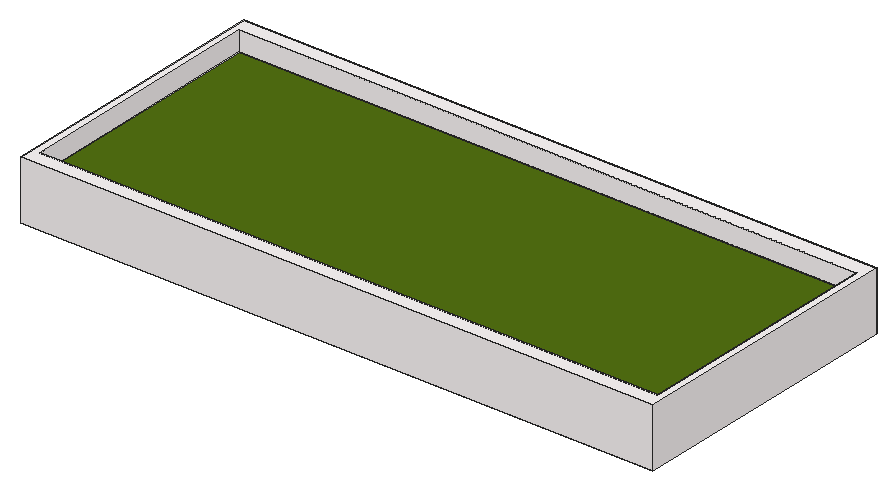
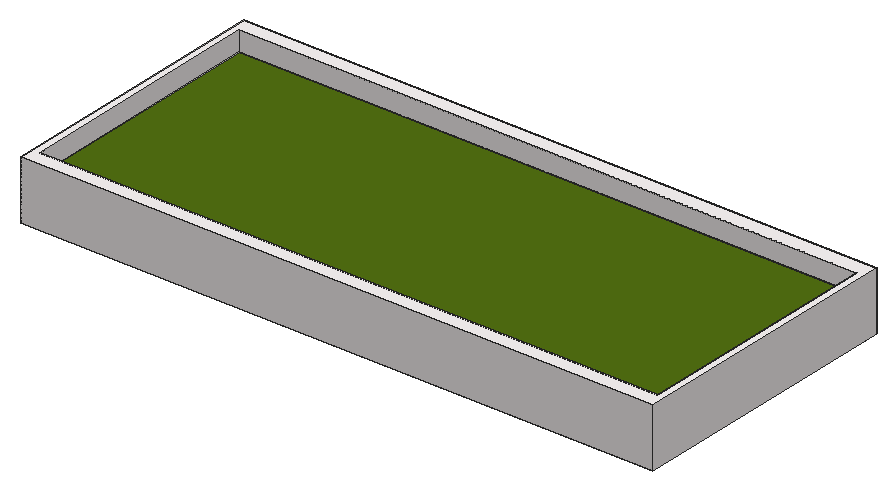
# SketchUp Ruby script. Lengths in inches.
U = 1.inch
M = Sketchup.active_model
def pt(a) = Geom::Point3d.new(a.map { |v| v * U })
def face(e, loops, mat)
  f = e.add_face(loops[0].map { |a| pt(a) })
  loops[1..].each { |l| e.add_face(l.map { |a| pt(a) }).erase! }
  f.material = f.back_material = mat if mat
  f
end
# faces: each face lists its corners as indices into pts; further lists are holes
def faces(e, pts, list, mat = nil) = list.each { |f| face(e, (f[0].is_a?(Array) ? f : [f]).map { |l| l.map { |i| pts[i] } }, mat) }
# xy, xz, yz: faces in a plane at the given z, y or x. An outline is a flat list of corners, or four numbers for a rectangle; further outlines are holes
def ring(l) = l.size == 4 ? [[l[0], l[1]], [l[2], l[1]], [l[2], l[3]], [l[0], l[3]]] : l.each_slice(2).to_a
def flat(e, list, mat, &to3) = list.each { |f| face(e, (f[0].is_a?(Array) ? f : [f]).map { |l| ring(l).map { |u, v| to3.(u, v) } }, mat) }
def xy(e, z, list, mat = nil) = flat(e, list, mat) { |x, y| [x, y, z] }
def xz(e, y, list, mat = nil) = flat(e, list, mat) { |x, z| [x, y, z] }
def yz(e, x, list, mat = nil) = flat(e, list, mat) { |y, z| [x, y, z] }
def lines(e, pts, list) = list.each { |a, b| e.add_line(pt(pts[a]), pt(pts[b])) }
# prism: a flat outline (further loops are holes) pulled along v
def prism(e, loops, v, mat = nil)
  f = face(e, loops, mat); d = Geom::Vector3d.new(v.map { |x| x * U })
  f.pushpull(f.normal.samedirection?(d) ? d.length : -d.length)
end
def box(e, o, s, mat = nil) = prism(e, [[o, [o[0] + s[0], o[1], o[2]], [o[0] + s[0], o[1] + s[1], o[2]], [o[0], o[1] + s[1], o[2]]]], [0, 0, s[2]], mat)
def at(x, y, z, deg = 0) = Geom::Transformation.translation(pt([x, y, z])) * Geom::Transformation.rotation(ORIGIN, Z_AXIS, deg.degrees)
def axes(o, x, y, z) = Geom::Transformation.new([*x, 0, *y, 0, *z, 0, *pt(o).to_a, 1])
def part(name) = M.definitions.add(name)
# library, detail: a bought-in or finely detailed component or shape, given as its bounding box
def library(name, o, s) = part(name).tap { |d| box(d.entities, o, s) }
def detail(e, o, s) = box(e.add_group.entities, o, s)
def put(e, d, t, mat = nil) = e.add_instance(d, t).tap { |i| i.material = mat if mat }
def group(e, t, mat = nil) = e.add_group.tap { |g| g.transformation = t; g.material = mat if mat }.entities
root = M.entities
M.materials.add("[0010_Snow]").color = [255, 250, 250]
M.materials.add("[Vegetation_Blur7]").color = [83, 114, 18]
xy(root,0,[[323.87,121.21,467.97,179.47]])
xy(root,0,[[[322.17,117.75,469.67,182.93],[323.87,121.21,467.97,179.47]]],"[0010_Snow]")
xy(root,9.13,[[323.87,121.21,467.97,179.47]],"[Vegetation_Blur7]")
xy(root,13.69,[[[322.17,117.75,469.67,182.93],[323.87,121.21,467.97,179.47]]],"[0010_Snow]")
xz(root,117.75,[[322.17,0,469.67,13.69]],"[0010_Snow]")
xz(root,121.21,[[323.87,0,467.97,9.13],[323.87,9.13,467.97,13.69]],"[0010_Snow]")
xz(root,179.47,[[323.87,0,467.97,9.13],[323.87,9.13,467.97,13.69]],"[0010_Snow]")
xz(root,182.93,[[322.17,0,469.67,13.69]],"[0010_Snow]")
yz(root,322.17,[[117.75,0,182.93,13.69]],"[0010_Snow]")
yz(root,323.87,[[121.21,0,179.47,9.13],[121.21,9.13,179.47,13.69]],"[0010_Snow]")
yz(root,467.97,[[121.21,0,179.47,9.13],[121.21,9.13,179.47,13.69]],"[0010_Snow]")
yz(root,469.67,[[117.75,0,182.93,13.69]],"[0010_Snow]")
